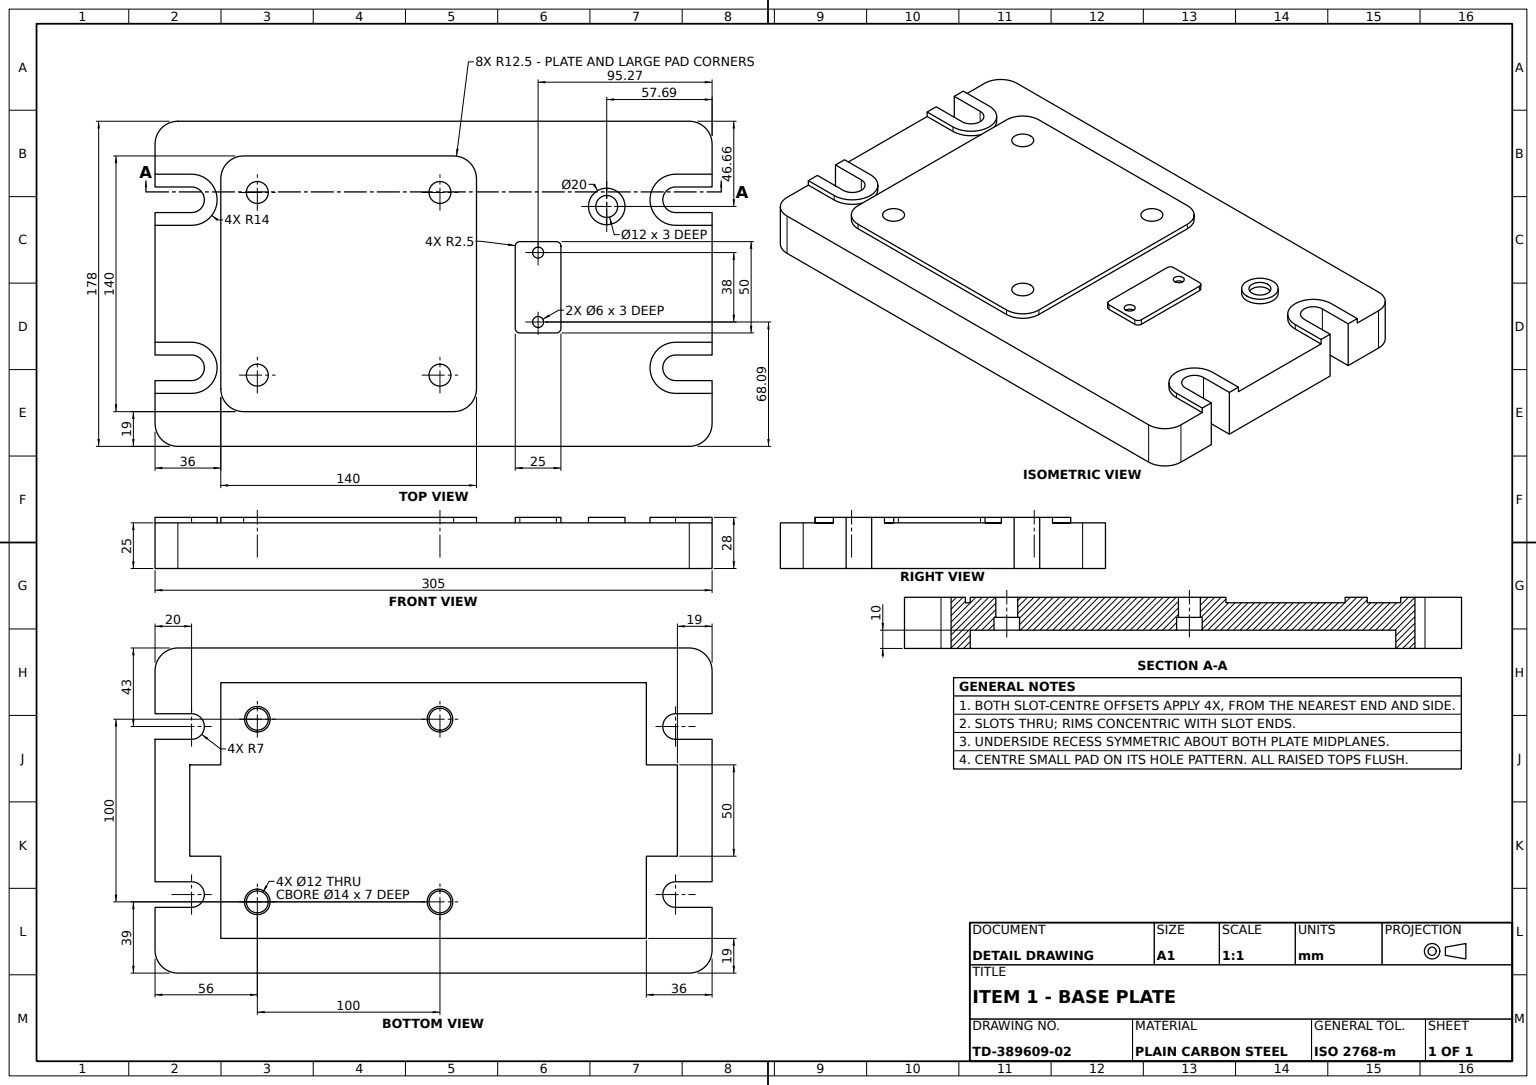
solid
v1 (57.228633,25,-14.091651)
v2 (57.228633,25,-20.091651)
e1 v1 v2 CIRCLE(AX(P(57.228633,25,-17.091651),D(0,-1,0),D(0,0,1)),3)
e2 v2 v1 CIRCLE(AX(P(57.228633,25,-17.091651),D(0,-1,0),D(0,0,1)),3)
face PLANE(AX(P(0,25,0),D(0,1,0),D(0,0,1))) [-e1 -e2]
v3 (-116.5,10,-70)
v4 (-116.5,0,-70)
e3 v3 v4 LINE
v5 (116.5,0,-70)
e4 v4 v5 LINE
v6 (116.5,10,-70)
e5 v6 v5 LINE
e6 v3 v6 LINE
face PLANE(AX(P(-116.5,10,-70),D(0,0,-1),D(-1,0,0))) rev [e3 e4 -e5 -e6]
v7 (152.5,28,39)
v8 (152.5,28,32)
e7 v7 v8 LINE
v9 (152.5,0,39)
e8 v7 v9 LINE
v10 (152.5,0,-39)
e9 v10 v9 LINE
v11 (152.5,28,-39)
e10 v11 v10 LINE
v12 (152.5,28,-32)
e11 v12 v11 LINE
v13 (152.5,25,-32)
e12 v12 v13 LINE
v14 (152.5,25,32)
e13 v13 v14 LINE
e14 v8 v14 LINE
face PLANE(AX(P(152.5,25,0),D(1,0,0),D(0,0,-1))) [-e7 e8 -e9 -e10 -e11 e12 e13 -e14]
v15 (3.5,10,-43)
v16 (3.5,10,-57)
e15 v15 v16 CIRCLE(AX(P(3.5,10,-50),D(0,1,0),D(0,0,-1)),7)
v17 (3.5,17,-43)
e16 v17 v15 LINE
v18 (3.5,17,-57)
e17 v17 v18 CIRCLE(AX(P(3.5,17,-50),D(0,1,0),D(0,0,-1)),7)
e18 v18 v16 LINE
face CYL(AX(P(3.5,17,-50),D(0,-1,0),D(0,0,-1)),7) rev [-e15 -e16 e17 e18]
v19 (67.228633,25,26.908349)
v20 (69.728633,25,24.408349)
e19 v19 v20 CIRCLE(AX(P(67.228633,25,24.408349),D(0,1,0),D(0,0,1)),2.5)
v21 (69.728633,28,24.408349)
e20 v21 v20 LINE
v22 (67.228633,28,26.908349)
e21 v22 v21 CIRCLE(AX(P(67.228633,28,24.408349),D(0,1,0),D(0,0,1)),2.5)
e22 v22 v19 LINE
face CYL(AX(P(67.228633,28,24.408349),D(0,-1,0),D(0,0,-1)),2.5) [e19 -e20 -e21 e22]
v23 (152.5,0,53)
v24 (132.5,0,53)
e23 v23 v24 LINE
v25 (132.5,28,53)
e24 v25 v24 LINE
v26 (152.5,28,53)
e25 v26 v25 LINE
e26 v26 v23 LINE
face PLANE(AX(P(0,25,53),D(0,0,1),D(1,0,0))) rev [e23 -e24 -e25 e26]
v27 (94.809461,28,-52.342377)
v28 (94.809461,28,-32.342377)
e27 v27 v28 CIRCLE(AX(P(94.809461,28,-42.342377),D(0,1,0),D(0,0,1)),10)
v29 (94.809461,25,-52.342377)
e28 v27 v29 LINE
v30 (94.809461,25,-32.342377)
e29 v29 v30 CIRCLE(AX(P(94.809461,25,-42.342377),D(0,1,0),D(0,0,1)),10)
e30 v28 v30 LINE
face CYL(AX(P(94.809461,28,-42.342377),D(0,-1,0),D(0,0,-1)),10) [-e27 e28 e29 -e30]
v31 (69.728633,25,-20.591651)
e31 v20 v31 LINE
v32 (69.728633,28,-20.591651)
e32 v32 v31 LINE
e33 v21 v32 LINE
face PLANE(AX(P(69.728633,28,-20.591651),D(-1,0,0),D(0,0,1))) rev [e20 e31 -e32 -e33]
v33 (132.5,28,-39)
v34 (132.5,0,-39)
e34 v33 v34 LINE
v35 (132.5,0,-53)
e35 v34 v35 CIRCLE(AX(P(132.5,0,-46),D(0,-1,0),D(0,0,1)),7)
v36 (132.5,28,-53)
e36 v36 v35 LINE
e37 v33 v36 CIRCLE(AX(P(132.5,28,-46),D(0,-1,0),D(0,0,-1)),7)
face CYL(AX(P(132.5,25,-46),D(0,-1,0),D(0,0,-1)),7) rev [e34 e35 -e36 -e37]
v37 (47.228633,28,-23.091651)
v38 (47.228633,25,-23.091651)
e38 v37 v38 LINE
v39 (44.728633,25,-20.591651)
e39 v38 v39 CIRCLE(AX(P(47.228633,25,-20.591651),D(0,1,0),D(0,0,1)),2.5)
v40 (44.728633,28,-20.591651)
e40 v40 v39 LINE
e41 v37 v40 CIRCLE(AX(P(47.228633,28,-20.591651),D(0,1,0),D(0,0,1)),2.5)
face CYL(AX(P(47.228633,28,-20.591651),D(0,-1,0),D(0,0,-1)),2.5) [e38 e39 -e40 -e41]
v41 (132.5,0,39)
e42 v41 v24 CIRCLE(AX(P(132.5,0,46),D(0,1,0),D(0,0,1)),7)
v42 (132.5,28,39)
e43 v42 v41 LINE
e44 v25 v42 CIRCLE(AX(P(132.5,28,46),D(0,-1,0),D(0,0,1)),7)
face CYL(AX(P(132.5,25,46),D(0,-1,0),D(0,0,-1)),7) rev [-e42 -e43 -e44 e24]
v43 (132.5,25,60)
v44 (152.5,25,60)
e45 v43 v44 LINE
v45 (152.5,28,60)
e46 v45 v44 LINE
v46 (132.5,28,60)
e47 v46 v45 LINE
e48 v46 v43 LINE
face PLANE(AX(P(152.5,28,60),D(0,0,-1),D(-1,0,0))) rev [e45 -e46 -e47 e48]
v47 (11,28,-70)
v48 (-104,28,-70)
e49 v47 v48 LINE
v49 (11,25,-70)
e50 v47 v49 LINE
v50 (-104,25,-70)
e51 v49 v50 LINE
e52 v48 v50 LINE
face PLANE(AX(P(-104,28,-70),D(0,0,1),D(1,0,0))) rev [-e49 e50 e51 -e52]
v51 (-96.5,10,43)
v52 (-96.5,10,57)
e53 v51 v52 CIRCLE(AX(P(-96.5,10,50),D(0,1,0),D(0,0,-1)),7)
v53 (-96.5,17,43)
e54 v53 v51 LINE
v54 (-96.5,17,57)
e55 v53 v54 CIRCLE(AX(P(-96.5,17,50),D(0,1,0),D(0,0,1)),7)
e56 v54 v52 LINE
face CYL(AX(P(-96.5,17,50),D(0,-1,0),D(0,0,-1)),7) rev [-e53 -e54 e55 e56]
v55 (133.5,10,25)
v56 (116.5,10,25)
e57 v55 v56 LINE
v57 (116.5,10,70)
e58 v56 v57 LINE
v58 (-116.5,10,70)
e59 v57 v58 LINE
v59 (-116.5,10,25)
e60 v58 v59 LINE
v60 (-133.5,10,25)
e61 v59 v60 LINE
v61 (-133.5,10,-25)
e62 v60 v61 LINE
v62 (-116.5,10,-25)
e63 v61 v62 LINE
e64 v62 v3 LINE
v63 (116.5,10,-25)
e65 v6 v63 LINE
v64 (133.5,10,-25)
e66 v63 v64 LINE
e67 v64 v55 LINE
v65 (3.5,10,57)
v66 (3.5,10,43)
e68 v65 v66 CIRCLE(AX(P(3.5,10,50),D(0,-1,0),D(0,0,-1)),7)
e69 v66 v65 CIRCLE(AX(P(3.5,10,50),D(0,-1,0),D(0,0,-1)),7)
v67 (-96.5,10,-57)
v68 (-96.5,10,-43)
e70 v67 v68 CIRCLE(AX(P(-96.5,10,-50),D(0,-1,0),D(0,0,-1)),7)
e71 v68 v67 CIRCLE(AX(P(-96.5,10,-50),D(0,-1,0),D(0,0,-1)),7)
e72 v52 v51 CIRCLE(AX(P(-96.5,10,50),D(0,1,0),D(0,0,-1)),7)
e73 v16 v15 CIRCLE(AX(P(3.5,10,-50),D(0,1,0),D(0,0,-1)),7)
face PLANE(AX(P(0,10,0),D(0,-1,0),D(0,0,-1))) [e57 e58 e59 e60 e61 e62 e63 e64 e6 e65 e66 e67] [-e68 -e69] [-e70 -e71] [e53 e72] [e73 e15]
v69 (-152.5,0,-39)
v70 (-132.5,0,-39)
e74 v69 v70 LINE
v71 (-152.5,28,-39)
e75 v71 v69 LINE
v72 (-132.5,28,-39)
e76 v72 v71 LINE
e77 v72 v70 LINE
face PLANE(AX(P(0,25,-39),D(0,0,-1),D(-1,0,0))) [-e74 -e75 -e76 e77]
v73 (44.728633,25,24.408349)
e78 v39 v73 LINE
v74 (44.728633,28,24.408349)
e79 v74 v73 LINE
e80 v40 v74 LINE
face PLANE(AX(P(44.728633,28,-20.591651),D(1,0,0),D(0,0,-1))) rev [e40 e78 -e79 -e80]
v75 (94.809461,25,-36.342377)
v76 (94.809461,25,-48.342377)
e81 v75 v76 CIRCLE(AX(P(94.809461,25,-42.342377),D(0,-1,0),D(0,0,1)),6)
v77 (94.809461,28,-48.342377)
e82 v77 v76 LINE
v78 (94.809461,28,-36.342377)
e83 v77 v78 CIRCLE(AX(P(94.809461,28,-42.342377),D(0,1,0),D(0,0,1)),6)
e84 v78 v75 LINE
face CYL(AX(P(94.809461,28,-42.342377),D(0,-1,0),D(0,0,-1)),6) rev [e81 -e82 e83 e84]
v79 (-133.5,0,25)
e85 v60 v79 LINE
v80 (-133.5,0,-25)
e86 v79 v80 LINE
e87 v61 v80 LINE
face PLANE(AX(P(-133.5,10,25),D(-1,0,0),D(0,0,1))) rev [-e62 e85 e86 -e87]
v81 (47.228633,25,26.908349)
e88 v73 v81 CIRCLE(AX(P(47.228633,25,24.408349),D(0,1,0),D(0,0,-1)),2.5)
v82 (47.228633,28,26.908349)
e89 v82 v81 LINE
e90 v74 v82 CIRCLE(AX(P(47.228633,28,24.408349),D(0,1,0),D(0,0,-1)),2.5)
face CYL(AX(P(47.228633,28,24.408349),D(0,-1,0),D(0,0,-1)),2.5) [e88 -e89 -e90 e79]
v83 (-152.5,28,32)
v84 (-152.5,28,39)
e91 v83 v84 LINE
v85 (-152.5,25,32)
e92 v83 v85 LINE
v86 (-152.5,25,-32)
e93 v86 v85 LINE
v87 (-152.5,28,-32)
e94 v87 v86 LINE
e95 v71 v87 LINE
v88 (-152.5,0,39)
e96 v69 v88 LINE
e97 v84 v88 LINE
face PLANE(AX(P(-152.5,25,0),D(1,0,0),D(0,0,-1))) rev [-e91 e92 -e93 -e94 -e95 e75 e96 -e97]
v89 (-96.5,17,-57)
v90 (-96.5,17,-43)
e98 v89 v90 CIRCLE(AX(P(-96.5,17,-50),D(0,-1,0),D(0,0,-1)),7)
e99 v89 v67 LINE
e100 v90 v68 LINE
face CYL(AX(P(-96.5,17,-50),D(0,-1,0),D(0,0,-1)),7) rev [-e98 e99 e70 -e100]
e101 v9 v41 LINE
v91 (152.5,0,76.5)
e102 v23 v91 LINE
v92 (140,0,89)
e103 v91 v92 CIRCLE(AX(P(140,0,76.5),D(0,-1,0),D(0,0,1)),12.5)
v93 (-140,0,89)
e104 v93 v92 LINE
v94 (-152.5,0,76.5)
e105 v93 v94 CIRCLE(AX(P(-140,0,76.5),D(0,-1,0),D(0,0,1)),12.5)
v95 (-152.5,0,53)
e106 v95 v94 LINE
v96 (-132.5,0,53)
e107 v95 v96 LINE
v97 (-132.5,0,39)
e108 v97 v96 CIRCLE(AX(P(-132.5,0,46),D(0,-1,0),D(0,0,1)),7)
e109 v88 v97 LINE
v98 (-132.5,0,-53)
e110 v70 v98 CIRCLE(AX(P(-132.5,0,-46),D(0,1,0),D(0,0,1)),7)
v99 (-152.5,0,-53)
e111 v99 v98 LINE
v100 (-152.5,0,-76.5)
e112 v100 v99 LINE
v101 (-140,0,-89)
e113 v100 v101 CIRCLE(AX(P(-140,0,-76.5),D(0,-1,0),D(0,0,1)),12.5)
v102 (140,0,-89)
e114 v101 v102 LINE
v103 (152.5,0,-76.5)
e115 v102 v103 CIRCLE(AX(P(140,0,-76.5),D(0,-1,0),D(0,0,1)),12.5)
v104 (152.5,0,-53)
e116 v103 v104 LINE
e117 v104 v35 LINE
e118 v10 v34 LINE
v105 (116.5,0,25)
v106 (116.5,0,70)
e119 v105 v106 LINE
v107 (133.5,0,25)
e120 v107 v105 LINE
v108 (133.5,0,-25)
e121 v108 v107 LINE
v109 (116.5,0,-25)
e122 v109 v108 LINE
e123 v5 v109 LINE
v110 (-116.5,0,-25)
e124 v110 v4 LINE
e125 v80 v110 LINE
v111 (-116.5,0,25)
e126 v111 v79 LINE
v112 (-116.5,0,70)
e127 v112 v111 LINE
e128 v106 v112 LINE
face PLANE(AX(P(0,0,0),D(0,1,0),D(0,0,1))) rev [e9 e101 e42 -e23 e102 e103 -e104 e105 -e106 e107 -e108 -e109 -e96 e74 e110 -e111 -e112 e113 e114 e115 e116 e117 -e35 -e118] [-e119 -e120 -e121 -e122 -e123 -e4 -e124 -e125 -e86 -e126 -e127 -e128]
v113 (23.5,28,-57.5)
e129 v113 v47 CIRCLE(AX(P(11,28,-57.5),D(0,1,0),D(0,0,1)),12.5)
v114 (23.5,25,-57.5)
e130 v113 v114 LINE
e131 v114 v49 CIRCLE(AX(P(11,25,-57.5),D(0,1,0),D(0,0,1)),12.5)
face CYL(AX(P(11,28,-57.5),D(0,-1,0),D(0,0,-1)),12.5) [-e129 e130 e131 -e50]
e132 v63 v109 LINE
face PLANE(AX(P(116.5,10,-25),D(1,0,0),D(0,0,-1))) rev [e123 -e132 -e65 e5]
v115 (3.5,17,56)
v116 (3.5,17,44)
e133 v115 v116 CIRCLE(AX(P(3.5,17,50),D(0,1,0),D(0,0,1)),6)
v117 (3.5,28,56)
e134 v117 v115 LINE
v118 (3.5,28,44)
e135 v117 v118 CIRCLE(AX(P(3.5,28,50),D(0,1,0),D(0,0,-1)),6)
e136 v118 v116 LINE
face CYL(AX(P(3.5,28,50),D(0,-1,0),D(0,0,-1)),6) rev [-e133 -e134 e135 e136]
v119 (132.5,28,32)
e137 v119 v46 CIRCLE(AX(P(132.5,28,46),D(0,1,0),D(0,0,1)),14)
e138 v45 v26 LINE
e139 v42 v7 LINE
e140 v8 v119 LINE
face PLANE(AX(P(132.5,28,46),D(0,1,0),D(0,0,1))) [e137 e47 e138 e25 e44 e139 e7 e140]
v120 (132.5,28,-60)
v121 (132.5,25,-60)
e141 v120 v121 LINE
v122 (152.5,28,-60)
e142 v122 v120 LINE
v123 (152.5,25,-60)
e143 v122 v123 LINE
e144 v123 v121 LINE
face PLANE(AX(P(152.5,28,-60),D(0,0,1),D(1,0,0))) rev [-e141 -e142 e143 e144]
e145 v56 v105 LINE
e146 v57 v106 LINE
face PLANE(AX(P(116.5,10,25),D(1,0,0),D(0,0,-1))) rev [e145 e119 -e146 -e58]
v124 (3.5,17,57)
v125 (3.5,17,43)
e147 v124 v125 CIRCLE(AX(P(3.5,17,50),D(0,-1,0),D(0,0,1)),7)
e148 v124 v65 LINE
e149 v125 v66 LINE
face CYL(AX(P(3.5,17,50),D(0,-1,0),D(0,0,-1)),7) rev [-e147 e148 e68 -e149]
v126 (-96.5,17,-44)
v127 (-96.5,17,-56)
e150 v126 v127 CIRCLE(AX(P(-96.5,17,-50),D(0,1,0),D(0,0,1)),6)
e151 v127 v126 CIRCLE(AX(P(-96.5,17,-50),D(0,1,0),D(0,0,1)),6)
e152 v90 v89 CIRCLE(AX(P(-96.5,17,-50),D(0,-1,0),D(0,0,-1)),7)
face PLANE(AX(P(-96.5,17,-50),D(0,1,0),D(0,0,-1))) rev [e150 e151] [e152 e98]
v128 (-140,25,-89)
e153 v101 v128 LINE
v129 (140,25,-89)
e154 v128 v129 LINE
e155 v129 v102 LINE
face PLANE(AX(P(0,25,-89),D(0,0,-1),D(-1,0,0))) [-e114 e153 e154 e155]
v130 (-132.5,25,32)
e156 v130 v85 LINE
v131 (-132.5,28,32)
e157 v131 v83 LINE
e158 v131 v130 LINE
face PLANE(AX(P(-152.5,28,32),D(0,0,1),D(1,0,0))) rev [e156 -e92 -e157 e158]
face CYL(AX(P(-96.5,17,-50),D(0,-1,0),D(0,0,-1)),7) rev [e100 e71 -e99 -e152]
v132 (-116.5,28,57.5)
v133 (-104,28,70)
e159 v132 v133 CIRCLE(AX(P(-104,28,57.5),D(0,1,0),D(0,0,1)),12.5)
v134 (-116.5,25,57.5)
e160 v132 v134 LINE
v135 (-104,25,70)
e161 v134 v135 CIRCLE(AX(P(-104,25,57.5),D(0,1,0),D(0,0,1)),12.5)
e162 v133 v135 LINE
face CYL(AX(P(-104,28,57.5),D(0,-1,0),D(0,0,-1)),12.5) [-e159 e160 e161 -e162]
e163 v30 v29 CIRCLE(AX(P(94.809461,25,-42.342377),D(0,1,0),D(0,0,1)),10)
e164 v28 v27 CIRCLE(AX(P(94.809461,28,-42.342377),D(0,1,0),D(0,0,1)),10)
face CYL(AX(P(94.809461,28,-42.342377),D(0,-1,0),D(0,0,-1)),10) [e30 e163 -e28 -e164]
e165 v18 v17 CIRCLE(AX(P(3.5,17,-50),D(0,1,0),D(0,0,-1)),7)
v136 (3.5,17,-44)
v137 (3.5,17,-56)
e166 v136 v137 CIRCLE(AX(P(3.5,17,-50),D(0,-1,0),D(0,0,1)),6)
e167 v137 v136 CIRCLE(AX(P(3.5,17,-50),D(0,-1,0),D(0,0,1)),6)
face PLANE(AX(P(3.5,17,-50),D(0,1,0),D(0,0,-1))) rev [-e165 -e17] [-e166 -e167]
face CYL(AX(P(3.5,17,-50),D(0,-1,0),D(0,0,-1)),7) rev [-e73 -e18 e165 e16]
v138 (-152.5,28,-53)
v139 (-132.5,28,-53)
e168 v138 v139 LINE
e169 v139 v72 CIRCLE(AX(P(-132.5,28,-46),D(0,-1,0),D(0,0,1)),7)
v140 (-132.5,28,-32)
e170 v87 v140 LINE
v141 (-132.5,28,-60)
e171 v140 v141 CIRCLE(AX(P(-132.5,28,-46),D(0,1,0),D(0,0,1)),14)
v142 (-152.5,28,-60)
e172 v141 v142 LINE
e173 v142 v138 LINE
face PLANE(AX(P(-132.5,28,-46),D(0,1,0),D(0,0,1))) [e168 e169 e76 e95 e170 e171 e172 e173]
e174 v58 v112 LINE
face PLANE(AX(P(-116.5,10,70),D(0,0,1),D(1,0,0))) rev [e128 -e174 -e59 e146]
e175 v55 v107 LINE
face PLANE(AX(P(133.5,10,25),D(0,0,1),D(1,0,0))) rev [e120 -e145 -e57 e175]
v143 (67.228633,28,-23.091651)
e176 v32 v143 CIRCLE(AX(P(67.228633,28,-20.591651),D(0,1,0),D(0,0,-1)),2.5)
v144 (67.228633,25,-23.091651)
e177 v31 v144 CIRCLE(AX(P(67.228633,25,-20.591651),D(0,1,0),D(0,0,-1)),2.5)
e178 v143 v144 LINE
face CYL(AX(P(67.228633,28,-20.591651),D(0,-1,0),D(0,0,-1)),2.5) [-e176 e32 e177 -e178]
v145 (-96.5,28,-44)
e179 v145 v126 LINE
v146 (-96.5,28,-56)
e180 v146 v127 LINE
e181 v146 v145 CIRCLE(AX(P(-96.5,28,-50),D(0,1,0),D(0,0,1)),6)
face CYL(AX(P(-96.5,28,-50),D(0,-1,0),D(0,0,-1)),6) rev [e179 -e151 -e180 e181]
v147 (-132.5,28,39)
e182 v147 v97 LINE
v148 (-132.5,28,53)
e183 v148 v96 LINE
e184 v147 v148 CIRCLE(AX(P(-132.5,28,46),D(0,-1,0),D(0,0,-1)),7)
face CYL(AX(P(-132.5,25,46),D(0,-1,0),D(0,0,-1)),7) rev [e182 e108 -e183 -e184]
v149 (57.228633,28,17.908349)
v150 (57.228633,25,17.908349)
e185 v149 v150 LINE
v151 (57.228633,28,23.908349)
e186 v149 v151 CIRCLE(AX(P(57.228633,28,20.908349),D(0,1,0),D(0,0,1)),3)
v152 (57.228633,25,23.908349)
e187 v151 v152 LINE
e188 v152 v150 CIRCLE(AX(P(57.228633,25,20.908349),D(0,-1,0),D(0,0,1)),3)
face CYL(AX(P(57.228633,28,20.908349),D(0,-1,0),D(0,0,-1)),3) rev [-e185 e186 e187 e188]
v153 (-152.5,28,60)
v154 (-132.5,28,60)
e189 v153 v154 LINE
v155 (-152.5,25,60)
e190 v153 v155 LINE
v156 (-132.5,25,60)
e191 v155 v156 LINE
e192 v154 v156 LINE
face PLANE(AX(P(-152.5,28,60),D(0,0,-1),D(-1,0,0))) rev [-e189 e190 e191 -e192]
v157 (132.5,28,-32)
e193 v120 v157 CIRCLE(AX(P(132.5,28,-46),D(0,1,0),D(0,0,-1)),14)
e194 v157 v12 LINE
e195 v11 v33 LINE
v158 (152.5,28,-53)
e196 v36 v158 LINE
e197 v158 v122 LINE
face PLANE(AX(P(132.5,28,-46),D(0,-1,0),D(0,0,-1))) rev [e142 e193 e194 e11 e195 e37 e196 e197]
v159 (-152.5,25,-60)
e198 v142 v159 LINE
v160 (-152.5,25,-76.5)
e199 v160 v159 LINE
e200 v160 v100 LINE
e201 v138 v99 LINE
face PLANE(AX(P(-152.5,25,0),D(1,0,0),D(0,0,-1))) rev [e198 -e199 e200 e112 -e201 -e173]
v161 (152.5,25,-76.5)
e202 v161 v123 LINE
e203 v158 v104 LINE
e204 v103 v161 LINE
face PLANE(AX(P(152.5,25,0),D(1,0,0),D(0,0,-1))) [e202 -e143 -e197 e203 -e116 e204]
e205 v78 v77 CIRCLE(AX(P(94.809461,28,-42.342377),D(0,1,0),D(0,0,1)),6)
face PLANE(AX(P(94.809461,28,-42.342377),D(0,1,0),D(0,0,1))) [-e83 -e205] [e27 e164]
face PLANE(AX(P(0,25,-53),D(0,0,1),D(1,0,0))) [e36 -e117 -e203 -e196]
e206 v59 v111 LINE
face PLANE(AX(P(-133.5,10,25),D(0,0,1),D(1,0,0))) rev [e126 -e85 -e61 e206]
v162 (57.228633,28,-14.091651)
e207 v162 v1 LINE
v163 (57.228633,28,-20.091651)
e208 v162 v163 CIRCLE(AX(P(57.228633,28,-17.091651),D(0,1,0),D(0,0,1)),3)
e209 v163 v2 LINE
face CYL(AX(P(57.228633,28,-17.091651),D(0,-1,0),D(0,0,-1)),3) rev [-e207 e208 e209 e2]
e210 v64 v108 LINE
face PLANE(AX(P(133.5,10,25),D(1,0,0),D(0,0,-1))) rev [-e67 e210 e121 -e175]
face PLANE(AX(P(133.5,10,-25),D(0,0,-1),D(-1,0,0))) rev [e122 -e210 -e66 e132]
v164 (-116.5,28,-57.5)
e211 v164 v132 LINE
v165 (-116.5,25,-57.5)
e212 v164 v165 LINE
e213 v165 v134 LINE
face PLANE(AX(P(-116.5,28,-57.5),D(1,0,0),D(0,0,-1))) rev [-e211 e212 e213 -e160]
v166 (152.5,25,76.5)
e214 v166 v91 LINE
e215 v44 v166 LINE
face PLANE(AX(P(152.5,25,0),D(1,0,0),D(0,0,-1))) [e214 -e102 -e26 -e138 e46 e215]
v167 (-152.5,25,76.5)
e216 v94 v167 LINE
e217 v155 v167 LINE
v168 (-152.5,28,53)
e218 v168 v153 LINE
e219 v168 v95 LINE
face PLANE(AX(P(-152.5,25,0),D(1,0,0),D(0,0,-1))) rev [e106 e216 -e217 -e190 -e218 e219]
v169 (132.5,25,32)
e220 v119 v169 LINE
e221 v169 v43 CIRCLE(AX(P(132.5,25,46),D(0,1,0),D(0,0,1)),14)
face CYL(AX(P(132.5,28,46),D(0,-1,0),D(0,0,-1)),14) [e220 e221 -e48 -e137]
e222 v161 v129 CIRCLE(AX(P(140,25,-76.5),D(0,1,0),D(0,0,1)),12.5)
face CYL(AX(P(140,25,-76.5),D(0,-1,0),D(0,0,-1)),12.5) [-e204 -e115 -e155 -e222]
e223 v150 v152 CIRCLE(AX(P(57.228633,25,20.908349),D(0,-1,0),D(0,0,1)),3)
e224 v151 v149 CIRCLE(AX(P(57.228633,28,20.908349),D(0,1,0),D(0,0,1)),3)
face CYL(AX(P(57.228633,28,20.908349),D(0,-1,0),D(0,0,-1)),3) rev [e185 e223 -e187 e224]
v170 (132.5,25,-32)
e225 v157 v170 LINE
e226 v170 v13 LINE
face PLANE(AX(P(152.5,28,-32),D(0,0,-1),D(-1,0,0))) rev [-e194 e225 e226 -e12]
v171 (-132.5,25,-60)
e227 v141 v171 LINE
e228 v171 v159 LINE
face PLANE(AX(P(-152.5,28,-60),D(0,0,1),D(1,0,0))) rev [-e198 -e172 e227 e228]
face PLANE(AX(P(0,25,0),D(0,1,0),D(0,0,1))) [-e223 -e188]
e229 v154 v131 CIRCLE(AX(P(-132.5,28,46),D(0,1,0),D(0,0,-1)),14)
e230 v84 v147 LINE
e231 v148 v168 LINE
face PLANE(AX(P(-132.5,28,46),D(0,-1,0),D(0,0,-1))) rev [e229 e157 e91 e230 e184 e231 e218 e189]
v172 (3.5,28,-56)
e232 v172 v137 LINE
v173 (3.5,28,-44)
e233 v172 v173 CIRCLE(AX(P(3.5,28,-50),D(0,1,0),D(0,0,-1)),6)
e234 v173 v136 LINE
face CYL(AX(P(3.5,28,-50),D(0,-1,0),D(0,0,-1)),6) rev [-e232 e233 e234 e166]
v174 (-140,25,89)
e235 v174 v93 LINE
e236 v167 v174 CIRCLE(AX(P(-140,25,76.5),D(0,1,0),D(0,0,1)),12.5)
face CYL(AX(P(-140,25,76.5),D(0,-1,0),D(0,0,-1)),12.5) [-e105 -e235 -e236 -e216]
e237 v76 v75 CIRCLE(AX(P(94.809461,25,-42.342377),D(0,-1,0),D(0,0,1)),6)
face PLANE(AX(P(0,25,0),D(0,1,0),D(0,0,1))) [-e81 -e237]
face PLANE(AX(P(0,25,39),D(0,0,-1),D(-1,0,0))) rev [e109 -e182 -e230 e97]
e238 v62 v110 LINE
face PLANE(AX(P(-133.5,10,-25),D(0,0,-1),D(-1,0,0))) rev [e87 e125 -e238 -e63]
e239 v125 v124 CIRCLE(AX(P(3.5,17,50),D(0,-1,0),D(0,0,1)),7)
face CYL(AX(P(3.5,17,50),D(0,-1,0),D(0,0,-1)),7) rev [-e239 e149 e69 -e148]
e240 v144 v38 LINE
e241 v143 v37 LINE
face PLANE(AX(P(47.228633,28,-23.091651),D(0,0,1),D(1,0,0))) rev [e178 e240 -e38 -e241]
v175 (-96.5,28,56)
v176 (-96.5,17,56)
e242 v175 v176 LINE
v177 (-96.5,28,44)
e243 v175 v177 CIRCLE(AX(P(-96.5,28,50),D(0,1,0),D(0,0,1)),6)
v178 (-96.5,17,44)
e244 v177 v178 LINE
e245 v178 v176 CIRCLE(AX(P(-96.5,17,50),D(0,-1,0),D(0,0,1)),6)
face CYL(AX(P(-96.5,28,50),D(0,-1,0),D(0,0,-1)),6) rev [-e242 e243 e244 e245]
e246 v139 v98 LINE
face CYL(AX(P(-132.5,25,-46),D(0,-1,0),D(0,0,-1)),7) rev [-e110 -e77 -e169 e246]
v179 (-132.5,25,-32)
e247 v179 v171 CIRCLE(AX(P(-132.5,25,-46),D(0,1,0),D(0,0,1)),14)
e248 v140 v179 LINE
face CYL(AX(P(-132.5,28,-46),D(0,-1,0),D(0,0,-1)),14) [e247 -e227 -e171 e248]
e249 v145 v146 CIRCLE(AX(P(-96.5,28,-50),D(0,1,0),D(0,0,1)),6)
e250 v177 v175 CIRCLE(AX(P(-96.5,28,50),D(0,1,0),D(0,0,1)),6)
e251 v173 v172 CIRCLE(AX(P(3.5,28,-50),D(0,1,0),D(0,0,-1)),6)
e252 v48 v164 CIRCLE(AX(P(-104,28,-57.5),D(0,1,0),D(0,0,-1)),12.5)
v180 (11,28,70)
e253 v133 v180 LINE
v181 (23.5,28,57.5)
e254 v180 v181 CIRCLE(AX(P(11,28,57.5),D(0,1,0),D(0,0,1)),12.5)
e255 v181 v113 LINE
e256 v118 v117 CIRCLE(AX(P(3.5,28,50),D(0,1,0),D(0,0,-1)),6)
face PLANE(AX(P(-104,28,57.5),D(0,1,0),D(0,0,1))) [-e181 -e249] [-e243 -e250] [-e233 -e251] [e129 e49 e252 e211 e159 e253 e254 e255] [-e256 -e135]
e257 v116 v115 CIRCLE(AX(P(3.5,17,50),D(0,1,0),D(0,0,1)),6)
face CYL(AX(P(3.5,28,50),D(0,-1,0),D(0,0,-1)),6) rev [e256 e134 -e257 -e136]
v182 (11,25,70)
e258 v180 v182 LINE
v183 (23.5,25,57.5)
e259 v182 v183 CIRCLE(AX(P(11,25,57.5),D(0,1,0),D(0,0,1)),12.5)
e260 v181 v183 LINE
face CYL(AX(P(11,28,57.5),D(0,-1,0),D(0,0,-1)),12.5) [-e254 e258 e259 -e260]
e261 v50 v165 CIRCLE(AX(P(-104,25,-57.5),D(0,1,0),D(0,0,-1)),12.5)
face CYL(AX(P(-104,28,-57.5),D(0,-1,0),D(0,0,-1)),12.5) [-e212 -e252 e52 e261]
face PLANE(AX(P(0,25,39),D(0,0,1),D(1,0,0))) [e43 -e101 -e8 -e139]
e262 v86 v179 LINE
face PLANE(AX(P(-152.5,28,-32),D(0,0,-1),D(-1,0,0))) rev [-e248 -e170 e94 e262]
v184 (140,25,89)
e263 v92 v184 LINE
e264 v174 v184 LINE
face PLANE(AX(P(0,25,89),D(0,0,-1),D(-1,0,0))) rev [e235 e104 e263 -e264]
e265 v156 v130 CIRCLE(AX(P(-132.5,25,46),D(0,1,0),D(0,0,-1)),14)
face CYL(AX(P(-132.5,28,46),D(0,-1,0),D(0,0,-1)),14) [e265 -e158 -e229 e192]
e266 v82 v22 LINE
e267 v163 v162 CIRCLE(AX(P(57.228633,28,-17.091651),D(0,1,0),D(0,0,1)),3)
face PLANE(AX(P(67.228633,28,-20.591651),D(0,-1,0),D(0,0,-1))) rev [-e186 -e224] [e21 e33 e176 e241 e41 e80 e90 e266] [-e208 -e267]
e268 v121 v170 CIRCLE(AX(P(132.5,25,-46),D(0,1,0),D(0,0,-1)),14)
face CYL(AX(P(132.5,28,-46),D(0,-1,0),D(0,0,-1)),14) [-e193 e141 e268 -e225]
face CYL(AX(P(3.5,28,-50),D(0,-1,0),D(0,0,-1)),6) rev [e232 e167 -e234 e251]
face PLANE(AX(P(0,25,-53),D(0,0,-1),D(-1,0,0))) rev [e201 e111 -e246 -e168]
e269 v183 v114 LINE
face PLANE(AX(P(23.5,28,-57.5),D(-1,0,0),D(0,0,1))) rev [e260 e269 -e130 -e255]
e270 v54 v53 CIRCLE(AX(P(-96.5,17,50),D(0,1,0),D(0,0,1)),7)
face CYL(AX(P(-96.5,17,50),D(0,-1,0),D(0,0,-1)),7) rev [e270 e54 -e72 -e56]
e271 v135 v182 LINE
face PLANE(AX(P(-104,28,70),D(0,0,-1),D(-1,0,0))) rev [e271 -e258 -e253 e162]
face CYL(AX(P(57.228633,28,-17.091651),D(0,-1,0),D(0,0,-1)),3) rev [e207 e1 -e209 e267]
face PLANE(AX(P(0,25,-39),D(0,0,1),D(1,0,0))) rev [-e34 -e195 e10 e118]
e272 v184 v166 CIRCLE(AX(P(140,25,76.5),D(0,1,0),D(0,0,1)),12.5)
face CYL(AX(P(140,25,76.5),D(0,1,0),D(0,0,1)),12.5) [-e263 -e103 -e214 -e272]
face CYL(AX(P(94.809461,28,-42.342377),D(0,-1,0),D(0,0,-1)),6) rev [e82 e237 -e84 e205]
e273 v14 v169 LINE
face PLANE(AX(P(152.5,28,32),D(0,0,1),D(1,0,0))) rev [-e140 e14 e273 -e220]
face PLANE(AX(P(0,25,53),D(0,0,-1),D(-1,0,0))) [-e219 -e231 e183 -e107]
face PLANE(AX(P(3.5,17,50),D(0,1,0),D(0,0,1))) rev [e239 e147] [e133 e257]
e274 v176 v178 CIRCLE(AX(P(-96.5,17,50),D(0,-1,0),D(0,0,1)),6)
face PLANE(AX(P(-96.5,17,50),D(0,1,0),D(0,0,1))) rev [-e270 -e55] [-e274 -e245]
face CYL(AX(P(-96.5,28,-50),D(0,-1,0),D(0,0,-1)),6) rev [e249 e180 -e150 -e179]
e275 v81 v19 LINE
face PLANE(AX(P(47.228633,28,26.908349),D(0,0,-1),D(-1,0,0))) rev [-e22 -e266 e89 e275]
e276 v128 v160 CIRCLE(AX(P(-140,25,-76.5),D(0,1,0),D(0,0,1)),12.5)
face PLANE(AX(P(0,25,0),D(0,1,0),D(0,0,1))) [-e163 -e29] [-e39 -e240 -e177 -e31 -e19 -e275 -e88 -e78] [-e247 -e262 e93 -e156 -e265 -e191 e217 e236 e264 e272 -e215 -e45 -e221 -e273 -e13 -e226 -e268 -e144 -e202 e222 -e154 e276 e199 -e228] [-e213 -e261 -e51 -e131 -e269 -e259 -e271 -e161]
face CYL(AX(P(-140,25,-76.5),D(0,1,0),D(0,0,1)),12.5) [-e113 -e200 -e276 -e153]
face CYL(AX(P(-96.5,28,50),D(0,-1,0),D(0,0,-1)),6) rev [e250 e242 e274 -e244]
face PLANE(AX(P(-116.5,10,-25),D(-1,0,0),D(0,0,1))) rev [e238 e124 -e3 -e64]
face PLANE(AX(P(-116.5,10,25),D(-1,0,0),D(0,0,1))) rev [e127 -e206 -e60 e174]
